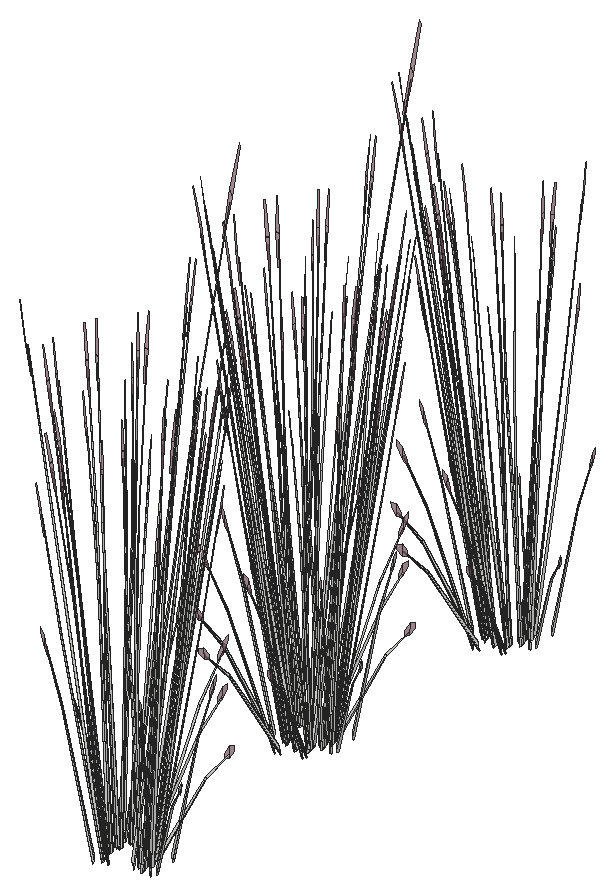
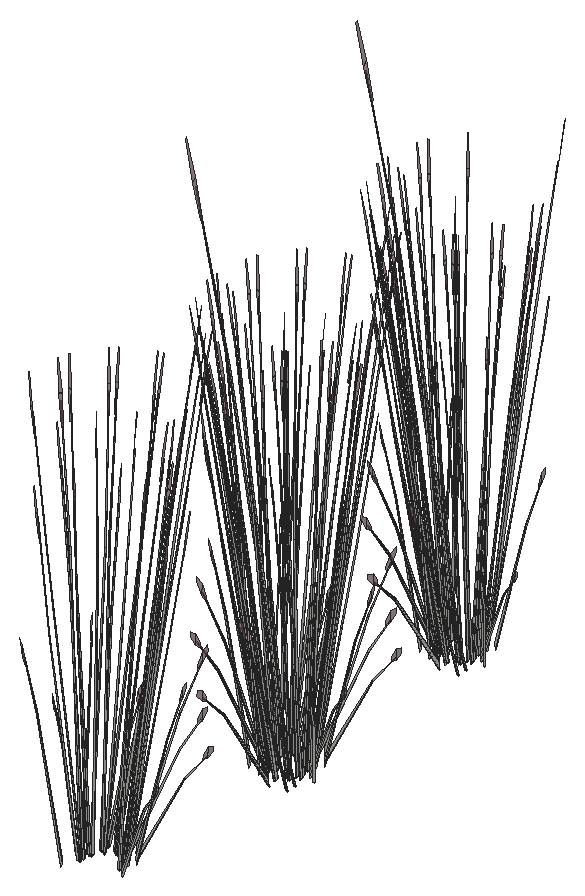
# SketchUp Ruby script. Lengths in inches.
U = 1.inch
M = Sketchup.active_model
def pt(a) = Geom::Point3d.new(a.map { |v| v * U })
def face(e, loops, mat)
  f = e.add_face(loops[0].map { |a| pt(a) })
  loops[1..].each { |l| e.add_face(l.map { |a| pt(a) }).erase! }
  f.material = f.back_material = mat if mat
  f
end
# faces: each face lists its corners as indices into pts; further lists are holes
def faces(e, pts, list, mat = nil) = list.each { |f| face(e, (f[0].is_a?(Array) ? f : [f]).map { |l| l.map { |i| pts[i] } }, mat) }
# xy, xz, yz: faces in a plane at the given z, y or x. An outline is a flat list of corners, or four numbers for a rectangle; further outlines are holes
def ring(l) = l.size == 4 ? [[l[0], l[1]], [l[2], l[1]], [l[2], l[3]], [l[0], l[3]]] : l.each_slice(2).to_a
def flat(e, list, mat, &to3) = list.each { |f| face(e, (f[0].is_a?(Array) ? f : [f]).map { |l| ring(l).map { |u, v| to3.(u, v) } }, mat) }
def xy(e, z, list, mat = nil) = flat(e, list, mat) { |x, y| [x, y, z] }
def xz(e, y, list, mat = nil) = flat(e, list, mat) { |x, z| [x, y, z] }
def yz(e, x, list, mat = nil) = flat(e, list, mat) { |y, z| [x, y, z] }
def lines(e, pts, list) = list.each { |a, b| e.add_line(pt(pts[a]), pt(pts[b])) }
# prism: a flat outline (further loops are holes) pulled along v
def prism(e, loops, v, mat = nil)
  f = face(e, loops, mat); d = Geom::Vector3d.new(v.map { |x| x * U })
  f.pushpull(f.normal.samedirection?(d) ? d.length : -d.length)
end
def box(e, o, s, mat = nil) = prism(e, [[o, [o[0] + s[0], o[1], o[2]], [o[0] + s[0], o[1] + s[1], o[2]], [o[0], o[1] + s[1], o[2]]]], [0, 0, s[2]], mat)
def at(x, y, z, deg = 0) = Geom::Transformation.translation(pt([x, y, z])) * Geom::Transformation.rotation(ORIGIN, Z_AXIS, deg.degrees)
def axes(o, x, y, z) = Geom::Transformation.new([*x, 0, *y, 0, *z, 0, *pt(o).to_a, 1])
def part(name) = M.definitions.add(name)
# library, detail: a bought-in or finely detailed component or shape, given as its bounding box
def library(name, o, s) = part(name).tap { |d| box(d.entities, o, s) }
def detail(e, o, s) = box(e.add_group.entities, o, s)
def put(e, d, t, mat = nil) = e.add_instance(d, t).tap { |i| i.material = mat if mat }
def group(e, t, mat = nil) = e.add_group.tap { |g| g.transformation = t; g.material = mat if mat }.entities
root = M.entities
M.materials.add("LightPink_Translucent").color = [144, 107, 117]
M.materials["LightPink_Translucent"].alpha = 0.75
c1 = part("blade")
p = [[2.15,0.21,22],[0,0.17,0],[0.09,0.45,0],[2.18,0.31,22],[2.29,0.31,22],[0.38,0.45,0],
  [2.48,0.24,33],[2.49,0.24,33],[2.48,0.22,33]]
faces(c1.entities,p,[[0,1,2,3],[4,5,2,3],[6,3,4,7],[8,0,3,6]])
c2 = part("seeds")
p = [[0.3,-0.1,1.38],[-0.01,-0.03,1.59],[-0.01,-0.03,0.03],[0.14,-0.07,-0.07],[0.29,-0.03,3],[0.15,0.01,3.11]]
faces(c2.entities,p,[[0,1,2,3],[1,0,4,5]],"LightPink_Translucent")
c3 = part("blade with seeds")
put(c3.entities,c1,at(0,0,0))
put(c3.entities,c2,axes([2.4,0.25,30.99],[1.5799,-0.05474,1.17369],[-0.12525,1.92788,0.29478],[-0.07173,-0.02425,1.56792]))
put(root,c3,axes([400.38,179.22,5.03],[-0.32648,-0.25715,-0.1216],[0.18809,-0.3724,-0.67495],[0.09224,-0.12945,1.02557]))
put(root,c3,axes([398.39,178.08,5.05],[0.05451,0.37564,0.35414],[-0.31161,0.09919,-0.4572],[-0.0837,-0.10765,0.87481]))
put(root,c3,axes([397.46,178.32,5.09],[0.29147,-0.34417,0.53763],[0.25138,0.3655,0.4433],[-0.13675,-0.06349,1.11249]))
put(root,c3,axes([401.18,179.11,4.71],[-0.0461,-0.00354,1.77383],[-0.19143,-0.37951,-0.16761],[0.07688,-0.12478,0.31391]))
put(root,c3,axes([397.59,178.32,4.73],[0.01777,-0.35463,0.0643],[0.26836,0.00972,0.50621],[-0.1028,-0.03711,0.77189]))
put(root,c3,axes([400.22,179.18,5.05],[-0.30722,0.06665,0.35414],[-0.08112,-0.381,-0.4572],[0.08804,-0.10234,0.87481]))
put(root,c3,axes([400.5,179.12,4.73],[0.2423,0.19613,0.0643],[-0.14107,0.2793,0.50621],[0.07768,-0.0903,0.77189]))
put(root,c3,axes([400.43,179.04,4.73],[0.08753,0.42921,0.48003],[-0.34336,0.07449,0.3958],[0.1012,-0.10094,0.9933]))
put(root,c3,axes([401.36,179.56,4.72],[0.04898,-0.07104,1.74944],[-0.06269,-0.43574,-0.27667],[0.12289,-0.08262,0.14031]))
put(root,c3,axes([397.22,177.86,4.71],[0.02617,0.04654,1.77383],[-0.12614,0.41836,-0.16761],[-0.12775,0.00303,0.31391]))
put(root,c3,axes([397.77,178.59,5.05],[0.20082,0.29199,0.35414],[-0.2293,0.2764,-0.4572],[-0.1165,-0.04206,0.87481]))
put(root,c3,axes([397.72,178.4,5.03],[-0.0189,0.47427,-0.1216],[-0.35781,-0.01296,-0.67495],[-0.13781,-0.03295,1.02557]))
put(root,c3,axes([400.39,180.22,5.03],[-0.17758,-0.42229,-0.1216],[0.31518,-0.20752,-0.67495],[0.13282,-0.05572,1.02557]))
put(root,c3,axes([400.27,180.09,5.05],[-0.29332,-0.1301,0.35414],[0.08555,-0.37955,-0.4572],[0.11809,-0.0348,0.87481]))
put(root,c3,axes([397.2,179.4,4.73],[0.09971,-0.42522,0.48003],[0.32782,0.1454,0.3958],[-0.12892,0.02555,0.9933]))
put(root,c3,axes([397.17,179.29,4.73],[-0.12963,-0.31798,0.0643],[0.23638,-0.15564,0.50621],[-0.1042,0.03071,0.77189]))
put(root,c3,axes([400.54,180.21,4.73],[0.12963,0.31798,0.0643],[-0.23638,0.15564,0.50621],[0.1042,-0.03071,0.77189]))
put(root,c3,axes([400.51,180.1,4.73],[-0.09971,0.42522,0.48003],[-0.32782,-0.1454,0.3958],[0.12892,-0.02555,0.9933]))
put(root,c3,axes([397.44,179.41,5.05],[0.29332,0.1301,0.35414],[-0.08555,0.37955,-0.4572],[-0.11809,0.0348,0.87481]))
put(root,c3,axes([401.1,181.48,4.71],[-0.03191,-0.04083,1.77383],[0.06981,-0.43764,-0.16761],[0.12571,-0.02796,0.31391]))
put(root,c3,axes([396.95,179.7,4.72],[-0.05763,0.06055,1.74944],[0.0049,0.44239,-0.27667],[-0.13211,0.05753,0.14031]))
put(root,c3,axes([397.32,179.28,5.03],[0.17758,0.42229,-0.1216],[-0.31518,0.20752,-0.67495],[-0.13282,0.05572,1.02557]))
put(root,c3,axes([399.99,181.1,5.03],[0.0189,-0.47427,-0.1216],[0.35781,0.01296,-0.67495],[0.13781,0.03295,1.02557]))
put(root,c3,axes([399.9375,180.91,5.05],[-0.20082,-0.29199,0.35414],[0.2293,-0.2764,-0.4572],[0.1165,0.04206,0.87481]))
put(root,c3,axes([400.31,180.8125,4.72],[0.07571,-0.00789,1.74944],[0.20767,-0.36231,-0.27667],[0.13467,0.04783,0.14031]))
put(root,c3,axes([397.28,180.46,4.73],[-0.08753,-0.42921,0.48003],[0.34336,-0.07449,0.3958],[-0.1012,0.10094,0.9933]))
put(root,c3,axes([397.21,180.375,4.73],[-0.2423,-0.19613,0.0643],[0.14107,-0.2793,0.50621],[-0.07768,0.0903,0.77189]))
put(root,c3,axes([397.49,180.32,5.05],[0.30722,-0.06665,0.35414],[0.08112,0.381,-0.4572],[-0.08804,0.10234,0.87481]))
put(root,c3,axes([396.31,180.15,4.71],[0.04504,0.01251,1.77383],[0.13934,0.41205,-0.16761],[-0.0922,0.10815,0.31391]))
put(root,c3,axes([400.12,181.18,4.73],[-0.01777,0.35463,0.0643],[-0.26836,-0.00972,0.50621],[0.1028,0.03711,0.77189]))
put(root,c3,axes([400.15,181.0625,4.73],[-0.26024,0.30729,0.48003],[-0.22444,-0.32634,0.3958],[0.1221,0.05668,0.9933]))
put(root,c3,axes([396.79,181.4,5.65],[0.31145,0.12449,-0.06488],[-0.0958,0.38314,-0.29416],[-0.05094,0.05817,0.97024]))
put(root,c3,axes([399.32,181.42,5.05],[-0.05451,-0.37564,0.35414],[0.31161,-0.09919,-0.4572],[0.0837,0.10765,0.87481]))
put(root,c3,axes([399.53,179.26,4.47],[-0.30498,-0.24231,1.38283],[0.32203,-0.37727,0.59665],[0.0984,0.22736,1.33663]))
put(root,c3,axes([397.33,180.28,5.03],[0.32648,0.25715,-0.1216],[-0.18809,0.3724,-0.67495],[-0.09224,0.12945,1.02557]))
put(root,c3,axes([399.29,181.61,5.03],[0.21031,-0.39918,-0.1216],[0.30457,0.22997,-0.67495],[0.10587,0.11278,1.02557]))
put(root,c3,axes([397.9,181.08,5.05],[0.23881,-0.24554,0.35414],[0.22606,0.28036,-0.4572],[-0.0344,0.14245,0.87481]))
put(root,c3,axes([399.01,181.95,4.71],[0.00104,-0.05646,1.77383],[0.30246,-0.2491,-0.16761],[0.10506,0.08891,0.31391]))
put(root,c3,axes([397.6875,181.3,4.73],[-0.29004,-0.02173,0.0643],[0.00795,-0.32812,0.50621],[-0.03035,0.12569,0.77189]))
put(root,c3,axes([397.78,181.33,4.73],[-0.25132,-0.3182,0.48003],[0.2669,-0.27442,0.3958],[-0.04636,0.14929,0.9933]))
put(root,c3,axes([398.57,181.48,5.05],[0.1064,-0.35863,0.35414],[0.31043,0.1046,-0.4572],[0.02846,0.14439,0.87481]))
put(root,c3,axes([399.37,181.76,4.73],[-0.16041,0.29625,0.0643],[-0.22843,-0.17248,0.50621],[0.07385,0.09498,0.77189]))
put(root,c3,axes([398.99,182.76,5.65],[0.2439,-0.26754,-0.06488],[0.22348,0.29302,-0.29416],[0.01573,0.08303,0.97024]))
put(root,c3,axes([399.44,181.68,4.73],[-0.35104,0.10702,0.48003],[-0.06092,-0.41983,0.3958],[0.08256,0.12373,0.9933]))
put(root,c3,axes([398.48,181.8,4.73],[-0.26007,0.1585,0.0643],[-0.12729,-0.28902,0.50621],[0.02512,0.1274,0.77189]))
put(root,c3,axes([396.96,181.35,4.72],[-0.00877,0.09229,1.74944],[0.24897,0.32105,-0.27667],[-0.06518,0.15182,0.14031]))
put(root,c3,axes([397.75,181.14,5.4],[0.3879,0.02311,-0.13498],[-0.0106,0.43749,-0.74919],[-0.02694,0.1685,1.13838]))
put(root,c3,axes([398.47,181.63,5.03],[0.34538,-0.21713,-0.1216],[0.16972,0.38536,-0.67495],[0.04557,0.16239,1.02557]))
put(root,c3,axes([398.57,181.77,5.0625],[-0.34777,-0.12192,0.53283],[0.11892,-0.40083,0.43934],[0.0209,0.15763,1.10256]))
put(root,c3,axes([396.93,182.3,4.71],[0.04004,-0.02816,1.77383],[0.33095,0.18728,-0.16761],[-0.00778,0.15594,0.31391]))
put(root,c3,axes([398.39,182.49,4.72],[0.04474,0.0751,1.74944],[0.36104,0.0295,-0.27667],[0.03631,0.16562,0.14031]))
put(root,c3,axes([397.68,196.9,4.72],[-0.05398,-0.06539,1.74944],[-0.36026,0.04145,-0.27667],[-0.0575,-0.15639,0.14031]))
put(root,c3,axes([399.29,197.7,4.72],[-0.00341,-0.09282,1.74944],[-0.28775,-0.26825,-0.27667],[0.04449,-0.16261,0.14031]))
put(root,c3,axes([399.22,197.36,4.71],[-0.03584,0.03562,1.77383],[-0.35118,-0.12018,-0.16761],[-0.01271,-0.15545,0.31391]))
put(root,c3,axes([397.31,196.68,4.71],[-0.00658,0.0559,1.77383],[-0.32474,0.20287,-0.16761],[-0.09556,-0.1037,0.31391]))
put(root,c3,axes([397.24,197.67,5.09],[0.39316,-0.11987,0.53763],[0.06823,0.47021,0.4433],[-0.09247,-0.13858,1.11249]))
put(root,c3,axes([398.125,197.76,4.73],[0.34777,0.12192,0.48003],[-0.11892,0.40083,0.3958],[-0.0209,-0.15763,0.9933]))
put(root,c3,axes([398.22,197.91,5.03],[-0.34538,0.21713,-0.1216],[-0.16972,-0.38536,-0.67495],[-0.04557,-0.16239,1.02557]))
put(root,c3,axes([398.94,198.39,5.03],[-0.3879,-0.02311,-0.1216],[0.0106,-0.43749,-0.67495],[0.02694,-0.1685,1.02557]))
put(root,c3,axes([398.22,197.73,4.73],[0.26007,-0.1585,0.0643],[0.12729,0.28902,0.50621],[-0.02512,-0.1274,0.77189]))
put(root,c3,axes([397.33,197.78,4.73],[0.16041,-0.29625,0.0643],[0.22843,0.17248,0.50621],[-0.07385,-0.09498,0.77189]))
put(root,c3,axes([398.12,198.06,5.05],[-0.1064,0.35863,0.35414],[-0.31043,-0.1046,-0.4572],[-0.02846,-0.14439,0.87481]))
put(root,c3,axes([398.91,198.21,4.73],[0.25132,0.3182,0.48003],[-0.2669,0.27442,0.3958],[0.04636,-0.14929,0.9933]))
put(root,c3,axes([397.4,197.74,5.43],[-0.23555,0.44708,-0.13619],[-0.34112,-0.25757,-0.75594],[-0.11858,-0.12631,1.14864]))
put(root,c3,axes([399.01,198.24,4.73],[0.29004,0.02173,0.0643],[-0.00795,0.32812,0.50621],[0.03035,-0.12569,0.77189]))
put(root,c3,axes([398.79,198.46,5.05],[-0.23881,0.24554,0.35414],[-0.22606,-0.28036,-0.4572],[0.0344,-0.14245,0.87481]))
put(root,c3,axes([396.5,197.62,4.72],[-0.07594,-0.00329,1.74944],[-0.24177,0.32918,-0.27667],[-0.129,-0.06726,0.14031]))
put(root,c3,axes([399.36,199.25,5.03],[-0.32648,-0.25715,-0.1216],[0.18809,-0.3724,-0.67495],[0.09224,-0.12945,1.02557]))
put(root,c3,axes([397.375,198.12,5.05],[0.05451,0.37564,0.35414],[-0.31161,0.09919,-0.4572],[-0.0837,-0.10765,0.87481]))
put(root,c3,axes([396.44,198.36,5.09],[0.29147,-0.34417,0.53763],[0.25138,0.3655,0.4433],[-0.13675,-0.06349,1.11249]))
put(root,c3,axes([400.17,199.14,4.71],[-0.0461,-0.00354,1.77383],[-0.19143,-0.37951,-0.16761],[0.07688,-0.12478,0.31391]))
put(root,c3,axes([396.57,198.36,4.73],[0.01777,-0.35463,0.0643],[0.26836,0.00972,0.50621],[-0.1028,-0.03711,0.77189]))
put(root,c3,axes([399.21,199.22,5.05],[-0.30722,0.06665,0.35414],[-0.08112,-0.381,-0.4572],[0.08804,-0.10234,0.87481]))
put(root,c3,axes([399.48,199.16,4.73],[0.2423,0.19613,0.0643],[-0.14107,0.2793,0.50621],[0.07768,-0.0903,0.77189]))
put(root,c3,axes([399.42,199.08,4.73],[0.08753,0.42921,0.48003],[-0.34336,0.07449,0.3958],[0.1012,-0.10094,0.9933]))
put(root,c3,axes([400.34,199.6,4.72],[0.04898,-0.07104,1.74944],[-0.06269,-0.43574,-0.27667],[0.12289,-0.08262,0.14031]))
put(root,c3,axes([396.2,197.9,4.71],[0.02617,0.04654,1.77383],[-0.12614,0.41836,-0.16761],[-0.12775,0.00303,0.31391]))
put(root,c3,axes([396.75,198.625,5.05],[0.20082,0.29199,0.35414],[-0.2293,0.2764,-0.4572],[-0.1165,-0.04206,0.87481]))
put(root,c3,axes([396.7,198.4375,5.03],[-0.0189,0.47427,-0.1216],[-0.35781,-0.01296,-0.67495],[-0.13781,-0.03295,1.02557]))
put(root,c3,axes([399.38,200.26,5.03],[-0.17758,-0.42229,-0.1216],[0.31518,-0.20752,-0.67495],[0.13282,-0.05572,1.02557]))
put(root,c3,axes([399.25,200.13,5.05],[-0.29332,-0.1301,0.35414],[0.08555,-0.37955,-0.4572],[0.11809,-0.0348,0.87481]))
put(root,c3,axes([396.18,199.4375,4.73],[0.09971,-0.42522,0.48003],[0.32782,0.1454,0.3958],[-0.12892,0.02555,0.9933]))
put(root,c3,axes([396.16,199.32,4.73],[-0.12963,-0.31798,0.0643],[0.23638,-0.15564,0.50621],[-0.1042,0.03071,0.77189]))
put(root,c3,axes([399.52,200.25,4.73],[0.12963,0.31798,0.0643],[-0.23638,0.15564,0.50621],[0.1042,-0.03071,0.77189]))
put(root,c3,axes([399.49,200.14,4.73],[-0.09971,0.42522,0.48003],[-0.32782,-0.1454,0.3958],[0.12892,-0.02555,0.9933]))
put(root,c3,axes([396.42,199.44,5.05],[0.29332,0.1301,0.35414],[-0.08555,0.37955,-0.4572],[-0.11809,0.0348,0.87481]))
put(root,c3,axes([400.08,201.51,4.71],[-0.03191,-0.04083,1.77383],[0.06981,-0.43764,-0.16761],[0.12571,-0.02796,0.31391]))
put(root,c3,axes([395.93,199.74,4.72],[-0.05763,0.06055,1.74944],[0.0049,0.44239,-0.27667],[-0.13211,0.05753,0.14031]))
put(root,c3,axes([396.3,199.31,5.03],[0.17758,0.42229,-0.1216],[-0.31518,0.20752,-0.67495],[-0.13282,0.05572,1.02557]))
put(root,c3,axes([398.98,201.14,5.03],[0.0189,-0.47427,-0.1216],[0.35781,0.01296,-0.67495],[0.13781,0.03295,1.02557]))
put(root,c3,axes([398.92,200.95,5.05],[-0.20082,-0.29199,0.35414],[0.2293,-0.2764,-0.4572],[0.1165,0.04206,0.87481]))
put(root,c3,axes([399.29,200.85,4.72],[0.07571,-0.00789,1.74944],[0.20767,-0.36231,-0.27667],[0.13467,0.04783,0.14031]))
put(root,c3,axes([396.26,200.5,4.73],[-0.08753,-0.42921,0.48003],[0.34336,-0.07449,0.3958],[-0.1012,0.10094,0.9933]))
put(root,c3,axes([396.19,200.41,4.73],[-0.2423,-0.19613,0.0643],[0.14107,-0.2793,0.50621],[-0.07768,0.0903,0.77189]))
put(root,c3,axes([396.47,200.35,5.05],[0.30722,-0.06665,0.35414],[0.08112,0.381,-0.4572],[-0.08804,0.10234,0.87481]))
put(root,c3,axes([395.29,200.18,4.71],[0.04504,0.01251,1.77383],[0.13934,0.41205,-0.16761],[-0.0922,0.10815,0.31391]))
put(root,c3,axes([399.11,201.21,4.73],[-0.01777,0.35463,0.0643],[-0.26836,-0.00972,0.50621],[0.1028,0.03711,0.77189]))
put(root,c3,axes([399.13,201.1,4.73],[-0.26024,0.30729,0.48003],[-0.22444,-0.32634,0.3958],[0.1221,0.05668,0.9933]))
put(root,c3,axes([395.78,201.43,5.65],[0.31145,0.12449,-0.06488],[-0.0958,0.38314,-0.29416],[-0.05094,0.05817,0.97024]))
put(root,c3,axes([398.3,201.46,5.05],[-0.05451,-0.37564,0.35414],[0.31161,-0.09919,-0.4572],[0.0837,0.10765,0.87481]))
put(root,c3,axes([398.51,199.3,4.47],[-0.30498,-0.24231,1.38283],[0.32203,-0.37727,0.59665],[0.0984,0.22736,1.33663]))
put(root,c3,axes([396.3125,200.32,5.03],[0.32648,0.25715,-0.1216],[-0.18809,0.3724,-0.67495],[-0.09224,0.12945,1.02557]))
put(root,c3,axes([398.27,201.65,5.03],[0.21031,-0.39918,-0.1216],[0.30457,0.22997,-0.67495],[0.10587,0.11278,1.02557]))
put(root,c3,axes([396.89,201.11,5.05],[0.23881,-0.24554,0.35414],[0.22606,0.28036,-0.4572],[-0.0344,0.14245,0.87481]))
put(root,c3,axes([398,201.98,4.71],[0.00104,-0.05646,1.77383],[0.30246,-0.2491,-0.16761],[0.10506,0.08891,0.31391]))
put(root,c3,axes([396.67,201.33,4.73],[-0.29004,-0.02173,0.0643],[0.00795,-0.32812,0.50621],[-0.03035,0.12569,0.77189]))
put(root,c3,axes([396.76,201.36,4.73],[-0.25132,-0.3182,0.48003],[0.2669,-0.27442,0.3958],[-0.04636,0.14929,0.9933]))
put(root,c3,axes([397.56,201.52,5.05],[0.1064,-0.35863,0.35414],[0.31043,0.1046,-0.4572],[0.02846,0.14439,0.87481]))
put(root,c3,axes([398.35,201.8,4.73],[-0.16041,0.29625,0.0643],[-0.22843,-0.17248,0.50621],[0.07385,0.09498,0.77189]))
put(root,c3,axes([397.98,202.8,5.65],[0.2439,-0.26754,-0.06488],[0.22348,0.29302,-0.29416],[0.01573,0.08303,0.97024]))
put(root,c3,axes([398.42,201.71,4.73],[-0.35104,0.10702,0.48003],[-0.06092,-0.41983,0.3958],[0.08256,0.12373,0.9933]))
put(root,c3,axes([397.46,201.84,4.73],[-0.26007,0.1585,0.0643],[-0.12729,-0.28902,0.50621],[0.02512,0.1274,0.77189]))
put(root,c3,axes([395.94,201.39,4.72],[-0.00877,0.09229,1.74944],[0.24897,0.32105,-0.27667],[-0.06518,0.15182,0.14031]))
put(root,c3,axes([396.74,201.18,5.4],[0.3879,0.02311,-0.13498],[-0.0106,0.43749,-0.74919],[-0.02694,0.1685,1.13838]))
put(root,c3,axes([397.45,201.67,5.03],[0.34538,-0.21713,-0.1216],[0.16972,0.38536,-0.67495],[0.04557,0.16239,1.02557]))
put(root,c3,axes([397.55,201.8125,5.0625],[-0.34777,-0.12192,0.53283],[0.11892,-0.40083,0.43934],[0.0209,0.15763,1.10256]))
put(root,c3,axes([395.91,202.33,4.71],[0.04004,-0.02816,1.77383],[0.33095,0.18728,-0.16761],[-0.00778,0.15594,0.31391]))
put(root,c3,axes([397.37,202.53,4.72],[0.04474,0.0751,1.74944],[0.36104,0.0295,-0.27667],[0.03631,0.16562,0.14031]))
put(root,c3,axes([399.16,215.73,4.72],[-0.05398,-0.06539,1.74944],[-0.36026,0.04145,-0.27667],[-0.0575,-0.15639,0.14031]))
put(root,c3,axes([400.78,216.53,4.72],[-0.00341,-0.09282,1.74944],[-0.28775,-0.26825,-0.27667],[0.04449,-0.16261,0.14031]))
put(root,c3,axes([400.7,216.19,4.71],[-0.03584,0.03562,1.77383],[-0.35118,-0.12018,-0.16761],[-0.01271,-0.15545,0.31391]))
put(root,c3,axes([398.79,215.51,4.71],[-0.00658,0.0559,1.77383],[-0.32474,0.20287,-0.16761],[-0.09556,-0.1037,0.31391]))
put(root,c3,axes([398.72,216.5,5.09],[0.39316,-0.11987,0.53763],[0.06823,0.47021,0.4433],[-0.09247,-0.13858,1.11249]))
put(root,c3,axes([399.61,216.59,4.73],[0.34777,0.12192,0.48003],[-0.11892,0.40083,0.3958],[-0.0209,-0.15763,0.9933]))
put(root,c3,axes([399.71,216.73,5.03],[-0.34538,0.21713,-0.1216],[-0.16972,-0.38536,-0.67495],[-0.04557,-0.16239,1.02557]))
put(root,c3,axes([400.42,217.22,5.03],[-0.3879,-0.02311,-0.1216],[0.0106,-0.43749,-0.67495],[0.02694,-0.1685,1.02557]))
put(root,c3,axes([399.7,216.56,4.73],[0.26007,-0.1585,0.0643],[0.12729,0.28902,0.50621],[-0.02512,-0.1274,0.77189]))
put(root,c3,axes([398.81,216.6,4.73],[0.16041,-0.29625,0.0643],[0.22843,0.17248,0.50621],[-0.07385,-0.09498,0.77189]))
put(root,c3,axes([399.6,216.89,5.05],[-0.1064,0.35863,0.35414],[-0.31043,-0.1046,-0.4572],[-0.02846,-0.14439,0.87481]))
put(root,c3,axes([400.39,217.04,4.73],[0.25132,0.3182,0.48003],[-0.2669,0.27442,0.3958],[0.04636,-0.14929,0.9933]))
put(root,c3,axes([398.88,216.57,5.43],[-0.23555,0.44708,-0.13619],[-0.34112,-0.25757,-0.75594],[-0.11858,-0.12631,1.14864]))
put(root,c3,axes([400.49,217.07,4.73],[0.29004,0.02173,0.0643],[-0.00795,0.32812,0.50621],[0.03035,-0.12569,0.77189]))
put(root,c3,axes([400.27,217.29,5.05],[-0.23881,0.24554,0.35414],[-0.22606,-0.28036,-0.4572],[0.0344,-0.14245,0.87481]))
put(root,c3,axes([397.98,216.44,4.72],[-0.07594,-0.00329,1.74944],[-0.24177,0.32918,-0.27667],[-0.129,-0.06726,0.14031]))
put(root,c3,axes([400.84,218.08,5.03],[-0.32648,-0.25715,-0.1216],[0.18809,-0.3724,-0.67495],[0.09224,-0.12945,1.02557]))
put(root,c3,axes([398.86,216.95,5.05],[0.05451,0.37564,0.35414],[-0.31161,0.09919,-0.4572],[-0.0837,-0.10765,0.87481]))
put(root,c3,axes([397.92,217.19,5.09],[0.29147,-0.34417,0.53763],[0.25138,0.3655,0.4433],[-0.13675,-0.06349,1.11249]))
put(root,c3,axes([401.65,217.97,4.71],[-0.0461,-0.00354,1.77383],[-0.19143,-0.37951,-0.16761],[0.07688,-0.12478,0.31391]))
put(root,c3,axes([398.05,217.1875,4.73],[0.01777,-0.35463,0.0643],[0.26836,0.00972,0.50621],[-0.1028,-0.03711,0.77189]))
put(root,c3,axes([400.6875,218.05,5.05],[-0.30722,0.06665,0.35414],[-0.08112,-0.381,-0.4572],[0.08804,-0.10234,0.87481]))
put(root,c3,axes([400.96,217.99,4.73],[0.2423,0.19613,0.0643],[-0.14107,0.2793,0.50621],[0.07768,-0.0903,0.77189]))
put(root,c3,axes([400.9,217.91,4.73],[0.08753,0.42921,0.48003],[-0.34336,0.07449,0.3958],[0.1012,-0.10094,0.9933]))
put(root,c3,axes([401.82,218.42,4.72],[0.04898,-0.07104,1.74944],[-0.06269,-0.43574,-0.27667],[0.12289,-0.08262,0.14031]))
put(root,c3,axes([397.68,216.72,4.71],[0.02617,0.04654,1.77383],[-0.12614,0.41836,-0.16761],[-0.12775,0.00303,0.31391]))
put(root,c3,axes([398.24,217.45,5.05],[0.20082,0.29199,0.35414],[-0.2293,0.2764,-0.4572],[-0.1165,-0.04206,0.87481]))
put(root,c3,axes([398.18,217.27,5.03],[-0.0189,0.47427,-0.1216],[-0.35781,-0.01296,-0.67495],[-0.13781,-0.03295,1.02557]))
put(root,c3,axes([400.86,219.09,5.03],[-0.17758,-0.42229,-0.1216],[0.31518,-0.20752,-0.67495],[0.13282,-0.05572,1.02557]))
put(root,c3,axes([400.73,218.96,5.05],[-0.29332,-0.1301,0.35414],[0.08555,-0.37955,-0.4572],[0.11809,-0.0348,0.87481]))
put(root,c3,axes([397.66,218.27,4.73],[0.09971,-0.42522,0.48003],[0.32782,0.1454,0.3958],[-0.12892,0.02555,0.9933]))
put(root,c3,axes([397.64,218.15,4.73],[-0.12963,-0.31798,0.0643],[0.23638,-0.15564,0.50621],[-0.1042,0.03071,0.77189]))
put(root,c3,axes([401,219.08,4.73],[0.12963,0.31798,0.0643],[-0.23638,0.15564,0.50621],[0.1042,-0.03071,0.77189]))
put(root,c3,axes([400.98,218.96,4.73],[-0.09971,0.42522,0.48003],[-0.32782,-0.1454,0.3958],[0.12892,-0.02555,0.9933]))
put(root,c3,axes([397.9,218.27,5.05],[0.29332,0.1301,0.35414],[-0.08555,0.37955,-0.4572],[-0.11809,0.0348,0.87481]))
put(root,c3,axes([401.5625,220.34,4.71],[-0.03191,-0.04083,1.77383],[0.06981,-0.43764,-0.16761],[0.12571,-0.02796,0.31391]))
put(root,c3,axes([397.41,218.57,4.72],[-0.05763,0.06055,1.74944],[0.0049,0.44239,-0.27667],[-0.13211,0.05753,0.14031]))
